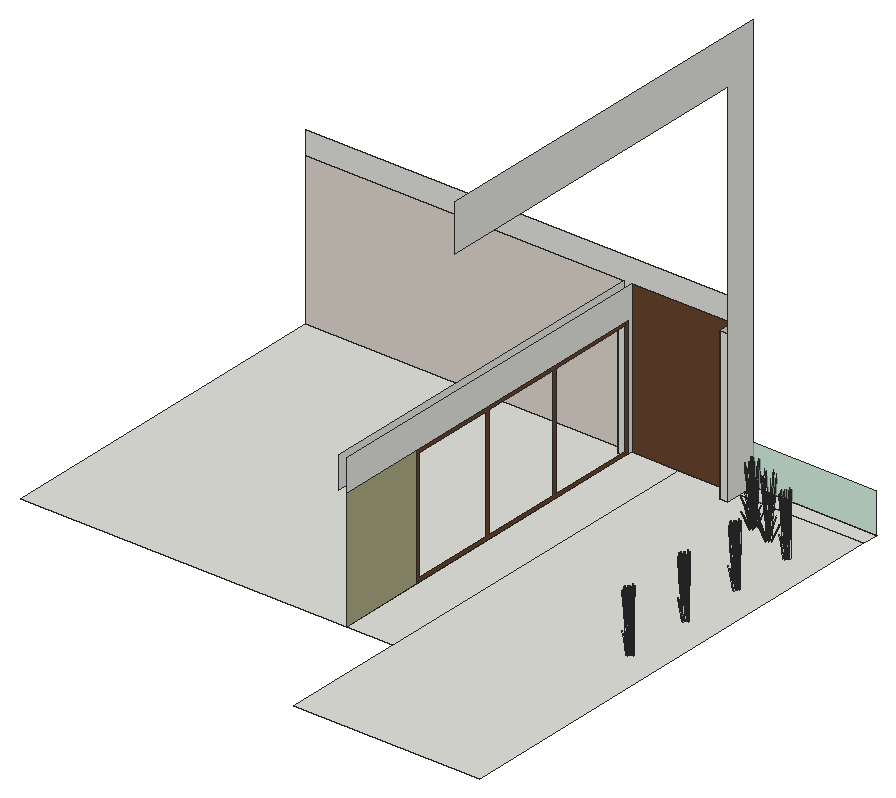
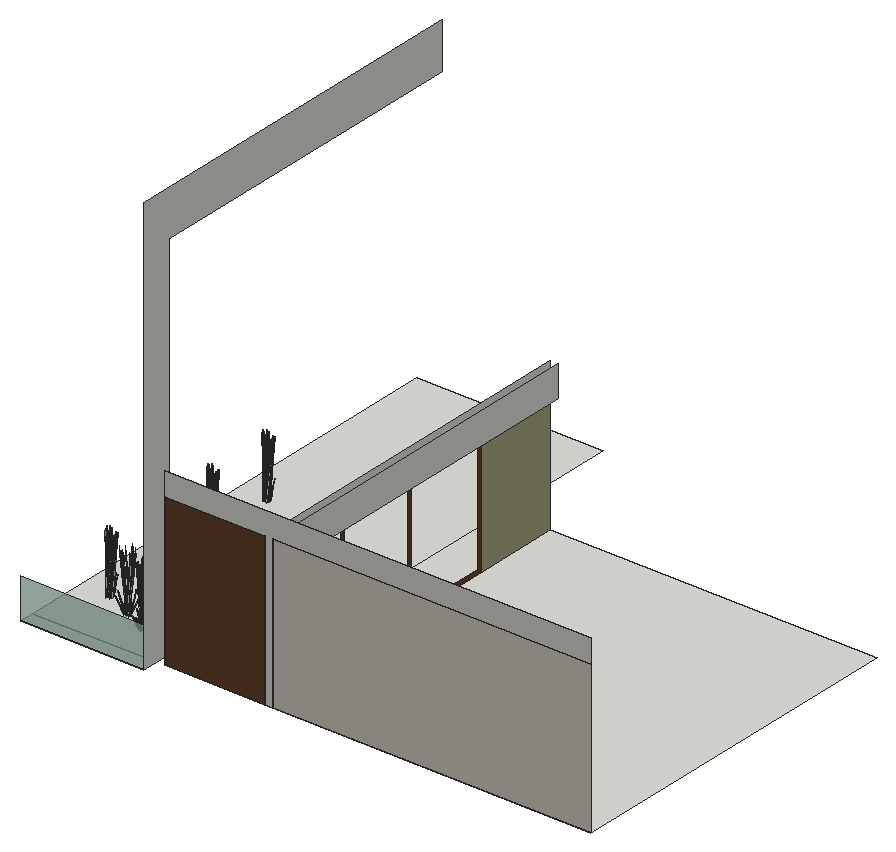
# SketchUp Ruby script. Lengths in inches.
U = 1.inch
M = Sketchup.active_model
def pt(a) = Geom::Point3d.new(a.map { |v| v * U })
def face(e, loops, mat)
  f = e.add_face(loops[0].map { |a| pt(a) })
  loops[1..].each { |l| e.add_face(l.map { |a| pt(a) }).erase! }
  f.material = f.back_material = mat if mat
  f
end
# faces: each face lists its corners as indices into pts; further lists are holes
def faces(e, pts, list, mat = nil) = list.each { |f| face(e, (f[0].is_a?(Array) ? f : [f]).map { |l| l.map { |i| pts[i] } }, mat) }
# xy, xz, yz: faces in a plane at the given z, y or x. An outline is a flat list of corners, or four numbers for a rectangle; further outlines are holes
def ring(l) = l.size == 4 ? [[l[0], l[1]], [l[2], l[1]], [l[2], l[3]], [l[0], l[3]]] : l.each_slice(2).to_a
def flat(e, list, mat, &to3) = list.each { |f| face(e, (f[0].is_a?(Array) ? f : [f]).map { |l| ring(l).map { |u, v| to3.(u, v) } }, mat) }
def xy(e, z, list, mat = nil) = flat(e, list, mat) { |x, y| [x, y, z] }
def xz(e, y, list, mat = nil) = flat(e, list, mat) { |x, z| [x, y, z] }
def yz(e, x, list, mat = nil) = flat(e, list, mat) { |y, z| [x, y, z] }
def lines(e, pts, list) = list.each { |a, b| e.add_line(pt(pts[a]), pt(pts[b])) }
# prism: a flat outline (further loops are holes) pulled along v
def prism(e, loops, v, mat = nil)
  f = face(e, loops, mat); d = Geom::Vector3d.new(v.map { |x| x * U })
  f.pushpull(f.normal.samedirection?(d) ? d.length : -d.length)
end
def box(e, o, s, mat = nil) = prism(e, [[o, [o[0] + s[0], o[1], o[2]], [o[0] + s[0], o[1] + s[1], o[2]], [o[0], o[1] + s[1], o[2]]]], [0, 0, s[2]], mat)
def at(x, y, z, deg = 0) = Geom::Transformation.translation(pt([x, y, z])) * Geom::Transformation.rotation(ORIGIN, Z_AXIS, deg.degrees)
def axes(o, x, y, z) = Geom::Transformation.new([*x, 0, *y, 0, *z, 0, *pt(o).to_a, 1])
def part(name) = M.definitions.add(name)
# library, detail: a bought-in or finely detailed component or shape, given as its bounding box
def library(name, o, s) = part(name).tap { |d| box(d.entities, o, s) }
def detail(e, o, s) = box(e.add_group.entities, o, s)
def put(e, d, t, mat = nil) = e.add_instance(d, t).tap { |i| i.material = mat if mat }
def group(e, t, mat = nil) = e.add_group.tap { |g| g.transformation = t; g.material = mat if mat }.entities
root = M.entities
M.materials.add("Carpet_2_1K").color = [170, 169, 131]
M.materials.add("LightPink_Translucent").color = [175, 214, 192]
M.materials["LightPink_Translucent"].alpha = 0.75
M.materials.add("ThomThom - Complexion1").color = [221, 214, 204]
M.materials.add("Wood_Veneer_15_1K").color = [103, 69, 45]
c1 = part("blade")
p = [[2.15,0.21,22],[0,0.17,0],[0.09,0.45,0],[2.18,0.31,22],[2.29,0.31,22],[0.38,0.45,0],
  [2.48,0.24,33],[2.49,0.24,33],[2.48,0.22,33]]
faces(c1.entities,p,[[0,1,2,3],[4,5,2,3],[6,3,4,7],[8,0,3,6]])
c2 = part("blade with seeds\#1")
put(c2.entities,c1,at(0,0,0))
c3 = part("seeds")
p = [[0.3,-0.1,1.38],[-0.01,-0.03,1.59],[-0.01,-0.03,0.03],[0.14,-0.07,-0.07],[0.29,-0.03,3],[0.15,0.01,3.11]]
faces(c3.entities,p,[[0,1,2,3],[1,0,4,5]],"LightPink_Translucent")
c4 = part("blade with seeds")
put(c4.entities,c1,at(0,0,0))
put(c4.entities,c3,axes([2.4,0.25,30.99],[1.5799,-0.05474,1.17369],[-0.12525,1.92788,0.29478],[-0.07173,-0.02425,1.56792]))
xy(root,138,[[366,222,510,222,510,594,414,594,414,582,408,582,408,594,366,594],[77.51,318,330,318,330,588,324,588,324,594,77.51,594],[330,318,366,594],[414,594,510,606]])
xz(root,582,[[408,138,414,255]])
xz(root,588,[[324,138,330,231]])
xz(root,594,[[324,138,330,138,330,255,408,255,408,273,77.51,273,77.51,255,324,255]])
xz(root,594,[[77.51,138,324,255]],"ThomThom - Complexion1")
xz(root,594,[[330,138,408,255]],"Wood_Veneer_15_1K")
xz(root,606,[[414,138,510,169.19]],"LightPink_Translucent")
yz(root,324,[[588,138,588,231,318,231,318,255,594,255,594,138]])
yz(root,330,[[591,138,594,138,594,255,318,255,318,231,591,231]])
yz(root,330,[[318,138,385.5,231]],"Carpet_2_1K")
yz(root,330,[[[385.5,138,588,138,588,141,456,141,456,228,517.5,228,517.5,141,520.5,141,520.5,228,588,228,588,231,385.5,231],[388.5,141,453,228]],[588,138,591,231]],"Wood_Veneer_15_1K")
yz(root,408,[[582,138,594,255]])
yz(root,414,[[582,138,606,138,606,462,318,462,318,426,582,426]])
put(root,c2,axes([443.42,567.05,138.04],[0.01373,0.08339,1.44662],[-0.15453,0.46112,-0.221],[-0.1289,-0.00774,0.24641]))
put(root,c2,axes([443.89,568.54,138.04],[0.0502,0.04815,1.44662],[0.10822,0.48665,-0.221],[-0.09845,0.11756,0.24641]))
put(root,c2,axes([444.07,565.01,138.04],[-0.03002,0.07441,1.44662],[-0.33536,0.19113,-0.221],[-0.09101,-0.12893,0.24641]))
put(root,c2,axes([443.68,567.14,138.56],[0.2186,0.34354,-0.03193],[-0.23941,0.31478,-0.14479],[-0.06784,0.02216,0.47756]))
put(root,c2,axes([444.14,567.82,138.76],[-0.38183,0.31082,0],[-0.21294,-0.52,-0.42336],[-0.0485,-0.11843,1.343]))
put(root,c2,axes([444.08,568.85,138.56],[0.31114,0.14341,-0.03193],[-0.09571,0.44138,-0.14479],[-0.05089,0.06702,0.47756]))
put(root,c2,axes([445.2,567.21,139],[-0.43479,0.05793,-0.23868],[-0.02629,-0.60335,-0.41019],[-0.05792,-0.10625,1.31016]))
put(root,c2,axes([445.65,567.49,139],[-0.18181,0.55986,-0.23868],[-0.38374,-0.26958,-0.41019],[-0.09422,0.01759,1.31016]))
put(root,c2,axes([445.5,569.08,138.76],[0,0.62163,0],[-0.42587,0,-0.42336],[-0.097,0,1.343]))
put(root,c2,axes([445.39,568.6,138.72],[0.32036,0.46241,0.25231],[-0.31699,0.46269,-0.29936],[-0.09098,0.01615,1.35263]))
put(root,c2,axes([446.06,567.35,138.8125],[-0.45152,-0.13176,-0.1922],[0.07871,-0.62475,0.4206],[-0.06235,0.10917,1.28336]))
put(root,c2,axes([444.24,565.53,138.76],[-0.38183,-0.31082,0],[0.21294,-0.52,-0.42336],[0.0485,-0.11843,1.343]))
put(root,c2,axes([445.75,564.31,138.4375],[0.04573,0.32019,1.16148],[-0.36399,0.05096,0.06648],[-0.05509,-0.22426,0.66092]))
put(root,c2,axes([445.43,563.72,138.67],[-0.24366,0.30821,-0.05322],[-0.22326,-0.33756,-0.24131],[-0.01572,-0.09565,0.79594]))
put(root,c2,axes([445.46,566.55,138.62],[-0.4409,0,0],[0,-0.62163,0],[0,0,1.47217]))
put(root,c2,axes([444.92,567.78,138.12],[0.15256,0.48933,1.05766],[-0.43772,0.15575,0.41096],[0.00728,-0.30048,1.20297]))
put(root,c2,axes([445.8,566.4,138.7],[-0.32797,0.46241,-0.0503],[-0.32817,-0.46269,0],[-0.01145,0.01615,1.4403]))
put(root,c2,axes([445.51,563.96,138.04],[-0.05785,0.02598,1.44662],[-0.33839,-0.1802,-0.221],[-0.00487,-0.18177,0.24641]))
put(root,c2,axes([445.45,569.32,138.04],[0.06005,-0.01261,1.44662],[0.31361,0.25416,-0.221],[-0.01581,0.18053,0.24641]))
put(root,c2,axes([445.14,566.51,139],[-0.25298,-0.50193,-0.23868],[0.35745,-0.33378,-0.41019],[0.0363,-0.12384,1.31016]))
put(root,c2,axes([446.05,567.07,139],[0.25298,0.50193,-0.23868],[-0.35745,0.33378,-0.41019],[-0.0363,0.12384,1.31016]))
put(root,c2,axes([445.56,566.13,138.62],[0,-0.5562,0],[0.39449,0,0],[0,0,1.46356]))
put(root,c2,axes([446.48,566.8125,138.62],[-0.32851,0.1622,0],[-0.11504,-0.46318,0],[0,0,1.26638]))
put(root,c2,axes([446.43,566.2,138.61],[-0.12929,-0.52192,-0.15749],[0.37242,-0.1834,0.00007],[-0.01429,-0.05761,1.42656]))
put(root,c2,axes([446.17,566.51,138.84],[-0.30669,0.48544,-0.20666],[-0.34439,-0.40848,0.45226],[0.03588,0.13072,1.37996]))
put(root,c2,axes([446.625,566.93,138.61],[-0.17107,0.50118,0],[-0.35546,-0.2412,0],[0,0,1.33477]))
put(root,c2,axes([445.63,566.24,138.69],[0.44068,0,-0.04624],[0,0.62163,0],[0.01385,0,1.47144]))
put(root,c2,axes([446.96,568.06,138.76],[0.38183,0.31082,0],[-0.21294,0.52,-0.42336],[-0.0485,0.11843,1.343]))
put(root,c2,axes([446.63,566.36,138.62],[0.17107,-0.50118,0],[0.35546,0.2412,0],[0,0,1.43523]))
put(root,c2,axes([447.01,566.16,138.61],[-0.38316,0.30694,-0.04218],[-0.21294,-0.52,0.42336],[0.03648,0.12814,1.34234]))
put(root,c2,axes([446.49,566.54,138.69],[0.43775,-0.21614,-0.04932],[0.15339,0.61757,0],[0.01529,-0.00755,1.41242]))
put(root,c2,axes([445.91,564.75,138.62],[-0.00305,0.62132,-0.04082],[-0.42587,0,0.4097],[0.09695,0.01953,1.29904]))
put(root,c2,axes([445.69,564.5,138.76],[0,-0.62163,0],[0.42587,0,-0.42336],[0.097,0,1.343]))
put(root,c2,axes([445.54,566.1,139],[0.18181,-0.55986,-0.23868],[0.38374,0.26958,-0.41019],[0.09422,-0.01759,1.31016]))
put(root,c2,axes([446,566.38,139],[0.43479,-0.05793,-0.23868],[0.02629,0.60335,-0.41019],[0.05792,0.10625,1.31016]))
put(root,c2,axes([446.8125,566.14,138.72],[0.12385,-0.62237,0.25231],[0.4427,0.1557,-0.29936],[0.05541,0.10301,1.35263]))
put(root,c2,axes([447.05,565.77,138.76],[0.38183,-0.31082,0],[0.21294,0.52,-0.42336],[0.0485,0.11843,1.343]))
put(root,c2,axes([447.18,565.27,138.04],[-0.05501,-0.03622,1.44662],[-0.16202,-0.45599,-0.221],[0.08385,-0.13824,0.24641]))
put(root,c2,axes([447.13,569.46,138.04],[0.03807,-0.06668,1.44662],[0.35272,-0.11307,-0.221],[0.07522,0.14779,0.24641]))
put(root,c2,axes([447.17,567.4,138.04],[-0.02073,-0.08046,1.44662],[0.11412,-0.48396,-0.221],[0.12863,-0.01415,0.24641]))
put(root,c4,axes([461.01,559.92,138.625],[0.01212,0.07018,1.60472],[-0.24435,0.36652,-0.24515],[-0.17356,-0.01847,0.27334]))
put(root,c4,axes([460.88,561.88,138.625],[0.06411,0.04449,1.60472],[0.1087,0.41223,-0.24515],[-0.14209,0.08791,0.27334]))
put(root,c4,axes([461.76,558.09,138.625],[-0.0463,0.05867,1.60472],[-0.46786,0.12648,-0.24515],[-0.11302,-0.11506,0.27334]))
put(root,c4,axes([462.08,561.24,139.11],[-0.11227,-0.38804,-0.2819],[0.44589,-0.11019,0.2819],[-0.08989,-0.04475,1.26466]))
put(root,c4,axes([462.87,560.41,139.28],[-0.28711,-0.37379,-0.40713],[0.43489,-0.26322,0.19594],[-0.09291,-0.04625,1.30716]))
put(root,c4,axes([463.48,560.68,139.28],[-0.519,0.02749,-0.40713],[-0.04694,-0.45634,0.19594],[-0.09291,0.04625,1.30716]))
put(root,c4,axes([463.92,561.68,139.11],[-0.44589,-0.11019,-0.2819],[0.11227,-0.38804,0.2819],[-0.08989,0.04475,1.26466]))
put(root,c4,axes([461.61,559.65,139.11],[0.33362,-0.27785,-0.2819],[0.33362,0.27785,0.2819],[0,-0.08949,1.26466]))
put(root,c4,axes([463.2,557.54,138.625],[-0.08017,0.01605,1.60472],[-0.44332,-0.18061,-0.24515],[0.00744,-0.15065,0.27334]))
put(root,c4,axes([462.83,559.82,139.28],[0.23189,-0.40128,-0.40713],[0.48183,0.19312,0.19594],[0,-0.0925,1.30716]))
put(root,c4,axes([462.86,561.92,138.625],[0.07735,-0.02423,1.60472],[0.46528,0.13338,-0.24515],[0.01361,0.15033,0.27334]))
put(root,c4,axes([464.06,560.36,139.28],[-0.23189,0.40128,-0.40713],[-0.48183,-0.19312,0.19594],[0,0.0925,1.30716]))
put(root,c4,axes([465.28,560.53,139.11],[-0.33362,0.27785,-0.2819],[-0.33362,-0.27785,0.2819],[0,0.08949,1.26466]))
put(root,c4,axes([462.97,558.5,139.11],[0.44589,0.11019,-0.2819],[-0.11227,0.38804,0.2819],[0.08989,-0.04475,1.26466]))
put(root,c4,axes([464.02,559.77,139.28],[0.28711,0.37379,-0.40713],[-0.43489,0.26322,0.19594],[0.09291,0.04625,1.30716]))
put(root,c4,axes([464.81,558.9375,139.11],[0.11227,0.38804,-0.2819],[-0.44589,0.11019,0.2819],[0.08989,0.04475,1.26466]))
put(root,c4,axes([465.16,558.31,138.625],[-0.07154,-0.03508,1.60472],[-0.18375,-0.39195,-0.24515],[0.12396,-0.10636,0.27334]))
put(root,c4,axes([464.91,561.9375,138.625],[0.03482,-0.06429,1.60472],[0.43839,-0.18935,-0.24515],[0.13291,0.098,0.27334]))
put(root,c4,axes([466.17,559.99,138.625],[-0.02498,-0.06761,1.60472],[0.17324,-0.39549,-0.24515],[0.17476,-0.00569,0.27334]))
put(root,c2,axes([485.02,399.27,138.66],[-0.31082,0.38183,0],[-0.52,-0.21294,-0.42336],[-0.11843,-0.0485,1.343]))
put(root,c2,axes([485.02,452.84,138.66],[-0.31082,0.38183,0],[-0.52,-0.21294,-0.42336],[-0.11843,-0.0485,1.343]))
put(root,c2,axes([485.02,502.05,138.66],[-0.31082,0.38183,0],[-0.52,-0.21294,-0.42336],[-0.11843,-0.0485,1.343]))
put(root,c2,axes([485.02,551.1,138.66],[-0.31082,0.38183,0],[-0.52,-0.21294,-0.42336],[-0.11843,-0.0485,1.343]))
put(root,c2,axes([484.23,396.39,138.46],[-0.14341,0.31114,-0.03193],[-0.44138,-0.09571,-0.14479],[-0.06702,-0.05089,0.47756]))
put(root,c2,axes([484.23,449.96,138.46],[-0.14341,0.31114,-0.03193],[-0.44138,-0.09571,-0.14479],[-0.06702,-0.05089,0.47756]))
put(root,c2,axes([484.23,499.17,138.46],[-0.14341,0.31114,-0.03193],[-0.44138,-0.09571,-0.14479],[-0.06702,-0.05089,0.47756]))
put(root,c2,axes([484.23,548.22,138.46],[-0.14341,0.31114,-0.03193],[-0.44138,-0.09571,-0.14479],[-0.06702,-0.05089,0.47756]))
put(root,c2,axes([483.99,397.8125,138.66],[-0.62163,0,0],[0,-0.42587,-0.42336],[0,-0.097,1.343]))
put(root,c2,axes([483.99,451.39,138.66],[-0.62163,0,0],[0,-0.42587,-0.42336],[0,-0.097,1.343]))
put(root,c2,axes([483.99,500.59,138.66],[-0.62163,0,0],[0,-0.42587,-0.42336],[0,-0.097,1.343]))
put(root,c2,axes([483.99,549.64,138.66],[-0.62163,0,0],[0,-0.42587,-0.42336],[0,-0.097,1.343]))
put(root,c2,axes([486,398.36,138.91],[-0.50193,0.25298,-0.23868],[-0.33378,-0.35745,-0.41019],[-0.12384,-0.0363,1.31016]))
put(root,c2,axes([486,451.9375,138.91],[-0.50193,0.25298,-0.23868],[-0.33378,-0.35745,-0.41019],[-0.12384,-0.0363,1.31016]))
put(root,c2,axes([486,501.15,138.91],[-0.50193,0.25298,-0.23868],[-0.33378,-0.35745,-0.41019],[-0.12384,-0.0363,1.31016]))
put(root,c2,axes([486,550.2,138.91],[-0.50193,0.25298,-0.23868],[-0.33378,-0.35745,-0.41019],[-0.12384,-0.0363,1.31016]))
put(root,c2,axes([484.47,397.7,138.63],[-0.46241,0.32036,0.25231],[-0.46269,-0.31699,-0.29936],[-0.01615,-0.09098,1.35263]))
put(root,c2,axes([484.47,451.27,138.63],[-0.46241,0.32036,0.25231],[-0.46269,-0.31699,-0.29936],[-0.01615,-0.09098,1.35263]))
put(root,c2,axes([484.47,500.48,138.63],[-0.46241,0.32036,0.25231],[-0.46269,-0.31699,-0.29936],[-0.01615,-0.09098,1.35263]))
put(root,c2,axes([484.47,549.53,138.63],[-0.46241,0.32036,0.25231],[-0.46269,-0.31699,-0.29936],[-0.01615,-0.09098,1.35263]))
put(root,c2,axes([486.5625,398.48,138.74],[-0.48544,-0.30669,-0.20666],[0.40848,-0.34439,0.45226],[-0.13072,0.03588,1.37996]))
put(root,c2,axes([486.5625,452.05,138.74],[-0.48544,-0.30669,-0.20666],[0.40848,-0.34439,0.45226],[-0.13072,0.03588,1.37996]))
put(root,c2,axes([486.5625,501.26,138.74],[-0.48544,-0.30669,-0.20666],[0.40848,-0.34439,0.45226],[-0.13072,0.03588,1.37996]))
put(root,c2,axes([486.5625,550.3125,138.74],[-0.48544,-0.30669,-0.20666],[0.40848,-0.34439,0.45226],[-0.13072,0.03588,1.37996]))
put(root,c2,axes([485.72,398.37,138.72],[0.13176,-0.45152,-0.1922],[0.62475,0.07871,0.4206],[-0.10917,-0.06235,1.28336]))
put(root,c2,axes([485.72,451.94,138.72],[0.13176,-0.45152,-0.1922],[0.62475,0.07871,0.4206],[-0.10917,-0.06235,1.28336]))
put(root,c2,axes([485.72,501.15,138.72],[0.13176,-0.45152,-0.1922],[0.62475,0.07871,0.4206],[-0.10917,-0.06235,1.28336]))
put(root,c2,axes([485.72,550.2,138.72],[0.13176,-0.45152,-0.1922],[0.62475,0.07871,0.4206],[-0.10917,-0.06235,1.28336]))
put(root,c2,axes([486.91,399.32,138.52],[-0.30694,-0.38316,-0.04218],[0.52,-0.21294,0.42336],[-0.12814,0.03648,1.34234]))
put(root,c2,axes([486.91,452.89,138.52],[-0.30694,-0.38316,-0.04218],[0.52,-0.21294,0.42336],[-0.12814,0.03648,1.34234]))
put(root,c2,axes([486.91,502.1,138.52],[-0.30694,-0.38316,-0.04218],[0.52,-0.21294,0.42336],[-0.12814,0.03648,1.34234]))
put(root,c2,axes([486.91,551.15,138.52],[-0.30694,-0.38316,-0.04218],[0.52,-0.21294,0.42336],[-0.12814,0.03648,1.34234]))
put(root,c2,axes([485.58,397.96,138.91],[-0.55986,-0.18181,-0.23868],[0.26958,-0.38374,-0.41019],[-0.01759,-0.09422,1.31016]))
put(root,c2,axes([485.58,451.54,138.91],[-0.55986,-0.18181,-0.23868],[0.26958,-0.38374,-0.41019],[-0.01759,-0.09422,1.31016]))
put(root,c2,axes([485.58,500.75,138.91],[-0.55986,-0.18181,-0.23868],[0.26958,-0.38374,-0.41019],[-0.01759,-0.09422,1.31016]))
put(root,c2,axes([485.58,549.8,138.91],[-0.55986,-0.18181,-0.23868],[0.26958,-0.38374,-0.41019],[-0.01759,-0.09422,1.31016]))
put(root,c2,axes([486.69,398.31,138.91],[0.05793,0.43479,-0.23868],[-0.60335,0.02629,-0.41019],[-0.10625,0.05792,1.31016]))
put(root,c2,axes([486.69,451.88,138.91],[0.05793,0.43479,-0.23868],[-0.60335,0.02629,-0.41019],[-0.10625,0.05792,1.31016]))
put(root,c2,axes([486.69,501.09,138.91],[0.05793,0.43479,-0.23868],[-0.60335,0.02629,-0.41019],[-0.10625,0.05792,1.31016]))
put(root,c2,axes([486.69,550.14,138.91],[0.05793,0.43479,-0.23868],[-0.60335,0.02629,-0.41019],[-0.10625,0.05792,1.31016]))
put(root,c2,axes([485.93,395.99,138.46],[-0.34354,0.2186,-0.03193],[-0.31478,-0.23941,-0.14479],[-0.02216,-0.06784,0.47756]))
put(root,c2,axes([485.93,449.57,138.46],[-0.34354,0.2186,-0.03193],[-0.31478,-0.23941,-0.14479],[-0.02216,-0.06784,0.47756]))
put(root,c2,axes([485.93,498.78,138.46],[-0.34354,0.2186,-0.03193],[-0.31478,-0.23941,-0.14479],[-0.02216,-0.06784,0.47756]))
put(root,c2,axes([485.93,547.83,138.46],[-0.34354,0.2186,-0.03193],[-0.31478,-0.23941,-0.14479],[-0.02216,-0.06784,0.47756]))
put(root,c2,axes([487.3,399.36,138.66],[0.31082,0.38183,0],[-0.52,0.21294,-0.42336],[-0.11843,0.0485,1.343]))
put(root,c2,axes([487.3,452.94,138.66],[0.31082,0.38183,0],[-0.52,0.21294,-0.42336],[-0.11843,0.0485,1.343]))
put(root,c2,axes([487.3,502.14,138.66],[0.31082,0.38183,0],[-0.52,0.21294,-0.42336],[-0.11843,0.0485,1.343]))
put(root,c2,axes([487.3,551.19,138.66],[0.31082,0.38183,0],[-0.52,0.21294,-0.42336],[-0.11843,0.0485,1.343]))
put(root,c2,axes([486.15,398.93,138.52],[-0.50118,-0.17107,0],[0.2412,-0.35546,0],[0,0,1.33477]))
put(root,c2,axes([486.15,452.51,138.52],[-0.50118,-0.17107,0],[0.2412,-0.35546,0],[0,0,1.33477]))
put(root,c2,axes([486.15,501.72,138.52],[-0.50118,-0.17107,0],[0.2412,-0.35546,0],[0,0,1.33477]))
put(root,c2,axes([486.15,550.77,138.52],[-0.50118,-0.17107,0],[0.2412,-0.35546,0],[0,0,1.33477]))
put(root,c2,axes([486.93,399.12,138.63],[0.62237,0.12385,0.25231],[-0.1557,0.4427,-0.29936],[-0.10301,0.05541,1.35263]))
put(root,c2,axes([486.93,452.7,138.63],[0.62237,0.12385,0.25231],[-0.1557,0.4427,-0.29936],[-0.10301,0.05541,1.35263]))
put(root,c2,axes([486.93,501.91,138.63],[0.62237,0.12385,0.25231],[-0.1557,0.4427,-0.29936],[-0.10301,0.05541,1.35263]))
put(root,c2,axes([486.93,550.95,138.63],[0.62237,0.12385,0.25231],[-0.1557,0.4427,-0.29936],[-0.10301,0.05541,1.35263]))
put(root,c2,axes([486.67,398.11,138.6],[-0.46241,-0.32797,-0.0503],[0.46269,-0.32817,0],[-0.01615,-0.01145,1.4403]))
put(root,c2,axes([486.67,451.68,138.6],[-0.46241,-0.32797,-0.0503],[0.46269,-0.32817,0],[-0.01615,-0.01145,1.4403]))
put(root,c2,axes([486.67,500.89,138.6],[-0.46241,-0.32797,-0.0503],[0.46269,-0.32817,0],[-0.01615,-0.01145,1.4403]))
put(root,c2,axes([486.67,549.94,138.6],[-0.46241,-0.32797,-0.0503],[0.46269,-0.32817,0],[-0.01615,-0.01145,1.4403]))
put(root,c2,axes([486.26,398.79,138.53],[-0.1622,-0.32851,0],[0.46318,-0.11504,0],[0,0,1.26638]))
put(root,c2,axes([486.26,452.36,138.53],[-0.1622,-0.32851,0],[0.46318,-0.11504,0],[0,0,1.26638]))
put(root,c2,axes([486.26,501.57,138.53],[-0.1622,-0.32851,0],[0.46318,-0.11504,0],[0,0,1.26638]))
put(root,c2,axes([486.26,550.62,138.53],[-0.1622,-0.32851,0],[0.46318,-0.11504,0],[0,0,1.26638]))
put(root,c2,axes([486.83,397.94,138.6],[0,0.44068,-0.04624],[-0.62163,0,0],[0,0.01385,1.47144]))
put(root,c2,axes([486.83,451.52,138.6],[0,0.44068,-0.04624],[-0.62163,0,0],[0,0.01385,1.47144]))
put(root,c2,axes([486.83,500.73,138.6],[0,0.44068,-0.04624],[-0.62163,0,0],[0,0.01385,1.47144]))
put(root,c2,axes([486.83,549.78,138.6],[0,0.44068,-0.04624],[-0.62163,0,0],[0,0.01385,1.47144]))
put(root,c2,axes([486.52,397.77,138.53],[0,-0.44089,0],[0.62163,0,0],[0,0,1.47217]))
put(root,c2,axes([486.52,451.34,138.53],[0,-0.44089,0],[0.62163,0,0],[0,0,1.47217]))
put(root,c2,axes([486.52,500.55,138.53],[0,-0.44089,0],[0.62163,0,0],[0,0,1.47217]))
put(root,c2,axes([486.52,549.6,138.53],[0,-0.44089,0],[0.62163,0,0],[0,0,1.47217]))
put(root,c2,axes([486.53,398.8,138.6],[0.21614,0.43775,-0.04932],[-0.61757,0.15339,0],[0.00755,0.01529,1.41242]))
put(root,c2,axes([486.53,452.37,138.6],[0.21614,0.43775,-0.04932],[-0.61757,0.15339,0],[0.00755,0.01529,1.41242]))
put(root,c2,axes([486.53,501.58,138.6],[0.21614,0.43775,-0.04932],[-0.61757,0.15339,0],[0.00755,0.01529,1.41242]))
put(root,c2,axes([486.53,550.63,138.6],[0.21614,0.43775,-0.04932],[-0.61757,0.15339,0],[0.00755,0.01529,1.41242]))
put(root,c2,axes([485.25,396.45,138.66],[-0.31082,-0.38183,0],[0.52,-0.21294,-0.42336],[0.11843,-0.0485,1.343]))
put(root,c2,axes([485.25,450.03,138.66],[-0.31082,-0.38183,0],[0.52,-0.21294,-0.42336],[0.11843,-0.0485,1.343]))
put(root,c2,axes([485.25,499.24,138.66],[-0.31082,-0.38183,0],[0.52,-0.21294,-0.42336],[0.11843,-0.0485,1.343]))
put(root,c2,axes([485.25,548.29,138.66],[-0.31082,-0.38183,0],[0.52,-0.21294,-0.42336],[0.11843,-0.0485,1.343]))
put(root,c2,axes([488.32,398.22,138.52],[-0.62132,-0.00305,-0.04082],[0,-0.42587,0.4097],[-0.01953,0.09695,1.29904]))
put(root,c2,axes([488.32,451.8,138.52],[-0.62132,-0.00305,-0.04082],[0,-0.42587,0.4097],[-0.01953,0.09695,1.29904]))
put(root,c2,axes([488.32,501.01,138.52],[-0.62132,-0.00305,-0.04082],[0,-0.42587,0.4097],[-0.01953,0.09695,1.29904]))
put(root,c2,axes([488.32,550.05,138.52],[-0.62132,-0.00305,-0.04082],[0,-0.42587,0.4097],[-0.01953,0.09695,1.29904]))
put(root,c2,axes([486.93,398.04,138.53],[0.34702,0.24613,0],[-0.34702,0.24613,0],[0,0,1.38858]))
put(root,c2,axes([486.93,451.61,138.53],[0.34702,0.24613,0],[-0.34702,0.24613,0],[0,0,1.38858]))
put(root,c2,axes([486.93,500.82,138.53],[0.34702,0.24613,0],[-0.34702,0.24613,0],[0,0,1.38858]))
put(root,c2,axes([486.93,549.87,138.53],[0.34702,0.24613,0],[-0.34702,0.24613,0],[0,0,1.38858]))
put(root,c2,axes([486.71,398.94,138.53],[0.50118,0.17107,0],[-0.2412,0.35546,0],[0,0,1.43523]))
put(root,c2,axes([486.71,452.51,138.53],[0.50118,0.17107,0],[-0.2412,0.35546,0],[0,0,1.43523]))
put(root,c2,axes([486.71,501.72,138.53],[0.50118,0.17107,0],[-0.2412,0.35546,0],[0,0,1.43523]))
put(root,c2,axes([486.71,550.77,138.53],[0.50118,0.17107,0],[-0.2412,0.35546,0],[0,0,1.43523]))
put(root,c2,axes([486.94,397.87,138.53],[0.5562,0,0],[0,0.39448,0],[0,0,1.46356]))
put(root,c2,axes([486.94,451.44,138.53],[0.5562,0,0],[0,0.39448,0],[0,0,1.46356]))
put(root,c2,axes([486.94,500.65,138.53],[0.5562,0,0],[0,0.39448,0],[0,0,1.46356]))
put(root,c2,axes([486.94,549.7,138.53],[0.5562,0,0],[0,0.39448,0],[0,0,1.46356]))
put(root,c2,axes([485.86,397.51,138.91],[-0.05793,-0.43479,-0.23868],[0.60335,-0.02629,-0.41019],[0.10625,-0.05792,1.31016]))
put(root,c2,axes([485.86,451.08,138.91],[-0.05793,-0.43479,-0.23868],[0.60335,-0.02629,-0.41019],[0.10625,-0.05792,1.31016]))
put(root,c2,axes([485.86,500.29,138.91],[-0.05793,-0.43479,-0.23868],[0.60335,-0.02629,-0.41019],[0.10625,-0.05792,1.31016]))
put(root,c2,axes([485.86,549.34,138.91],[-0.05793,-0.43479,-0.23868],[0.60335,-0.02629,-0.41019],[0.10625,-0.05792,1.31016]))
